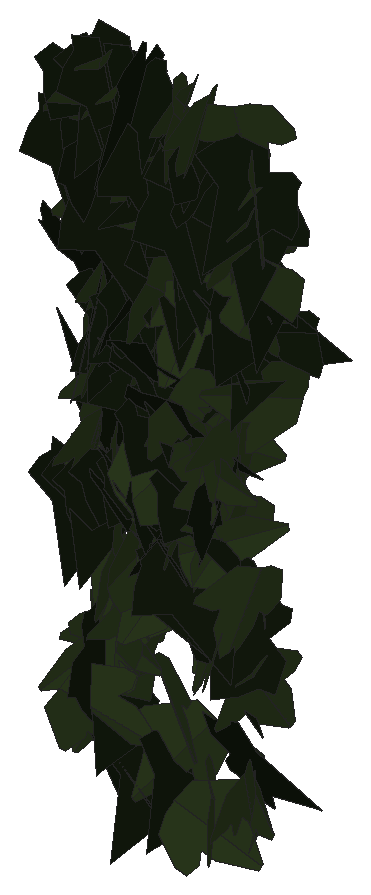
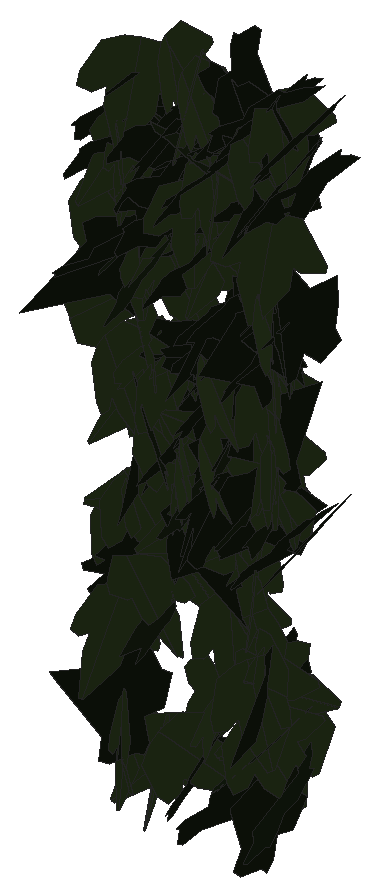
# SketchUp Ruby script. Lengths in inches.
U = 1.inch
M = Sketchup.active_model
def pt(a) = Geom::Point3d.new(a.map { |v| v * U })
def face(e, loops, mat)
  f = e.add_face(loops[0].map { |a| pt(a) })
  loops[1..].each { |l| e.add_face(l.map { |a| pt(a) }).erase! }
  f.material = f.back_material = mat if mat
  f
end
# faces: each face lists its corners as indices into pts; further lists are holes
def faces(e, pts, list, mat = nil) = list.each { |f| face(e, (f[0].is_a?(Array) ? f : [f]).map { |l| l.map { |i| pts[i] } }, mat) }
# xy, xz, yz: faces in a plane at the given z, y or x. An outline is a flat list of corners, or four numbers for a rectangle; further outlines are holes
def ring(l) = l.size == 4 ? [[l[0], l[1]], [l[2], l[1]], [l[2], l[3]], [l[0], l[3]]] : l.each_slice(2).to_a
def flat(e, list, mat, &to3) = list.each { |f| face(e, (f[0].is_a?(Array) ? f : [f]).map { |l| ring(l).map { |u, v| to3.(u, v) } }, mat) }
def xy(e, z, list, mat = nil) = flat(e, list, mat) { |x, y| [x, y, z] }
def xz(e, y, list, mat = nil) = flat(e, list, mat) { |x, z| [x, y, z] }
def yz(e, x, list, mat = nil) = flat(e, list, mat) { |y, z| [x, y, z] }
def lines(e, pts, list) = list.each { |a, b| e.add_line(pt(pts[a]), pt(pts[b])) }
# prism: a flat outline (further loops are holes) pulled along v
def prism(e, loops, v, mat = nil)
  f = face(e, loops, mat); d = Geom::Vector3d.new(v.map { |x| x * U })
  f.pushpull(f.normal.samedirection?(d) ? d.length : -d.length)
end
def box(e, o, s, mat = nil) = prism(e, [[o, [o[0] + s[0], o[1], o[2]], [o[0] + s[0], o[1] + s[1], o[2]], [o[0], o[1] + s[1], o[2]]]], [0, 0, s[2]], mat)
def at(x, y, z, deg = 0) = Geom::Transformation.translation(pt([x, y, z])) * Geom::Transformation.rotation(ORIGIN, Z_AXIS, deg.degrees)
def axes(o, x, y, z) = Geom::Transformation.new([*x, 0, *y, 0, *z, 0, *pt(o).to_a, 1])
def part(name) = M.definitions.add(name)
# library, detail: a bought-in or finely detailed component or shape, given as its bounding box
def library(name, o, s) = part(name).tap { |d| box(d.entities, o, s) }
def detail(e, o, s) = box(e.add_group.entities, o, s)
def put(e, d, t, mat = nil) = e.add_instance(d, t).tap { |i| i.material = mat if mat }
def group(e, t, mat = nil) = e.add_group.tap { |g| g.transformation = t; g.material = mat if mat }.entities
root = M.entities
M.materials.add("efeu1").color = [18, 25, 13]
M.materials.add("efeu2").color = [43, 57, 29]
c1 = part("ivyleaf_10")
p = [[0,0.5,-0.03],[-0.0625,2.02,-0.43],[-0.19,2.01,-0.46],[-0.54,1.05,-0.29],[-0.52,0.625,-0.18],[-0.83,0.76,-0.28],
  [-1.16,0.64,-0.33],[-1.15,0.33,-0.24],[-0.77,-0.39,0.02],[-0.3,-0.51,0.16],[0.04,-0.48,0.23],[-0.02,2.01,-0.4375],
  [-0.06,2.01,-0.43],[0.04,-0.49,0.23],[0.67,-0.49,0.14],[1.38,0.36,-0.2],[1.375,0.51,-0.24],[0.81,0.65,-0.19],
  [0.62,0.59,-0.15],[0.6,1.09,-0.28],[0.5,1.23,-0.31]]
faces(c1.entities,p,[[0,1,2,3,4,5,6,7,8,9,10],[11,12,0,13,14,15,16,17,18,19,20]],"efeu2")
c2 = part("ivyleaf_9")
p = [[1.54,2.16,1.25],[1.36,2.04,1.19],[-0.21,0.99,0.68],[-0.71,1.11,0.82],[-0.85,0.86,0.67],[-0.8,0.17,0.21],
  [-0.9,-0.01,0.1],[-0.67,-0.16,-0.02],[-0.08,-0.08,-0.05],[-0.03,-0.6,-0.4],[0.65,-0.88,-0.66],[0.83,-0.6,-0.49],
  [1.29,-0.42,-0.43],[1.8125,-0.07,-0.26],[1.21,0.44,0.15]]
faces(c2.entities,p,[[0,1,2,3,4,5,6,7,8,9,10,11,12,13,14]],"efeu1")
put(root,c1,axes([19.36,223.77,215.16],[-0.23772,-0.16251,-0.40876],[0.39056,0.13578,-0.28112],[0.20237,-0.45294,0.06239]))
put(root,c2,axes([21.28,224.3,220.56],[-0.0985,-0.38619,0.30192],[0.08114,-0.31655,-0.37843],[0.48344,-0.02556,0.12503]))
put(root,c2,axes([20.67,224.1,221.75],[0.00218,-0.49525,-0.06872],[0.00356,0.06873,-0.49524],[0.49998,0.00167,0.00383]))
put(root,c2,axes([19.62,223.89,217.87],[0.43761,-0.23745,-0.04594],[-0.03954,0.02345,-0.49788],[0.2386,0.43939,0.00174]))
put(root,c2,axes([20.26,223.86,219.03],[0.41406,-0.10025,0.26174],[0.25775,-0.04721,-0.42583],[0.11009,0.48757,0.01258]))
put(root,c2,axes([18.99,224.28,217.52],[-0.01258,-0.43972,0.23767],[0.03524,-0.23794,-0.43834],[0.4986,0.00572,0.03698]))
put(root,c1,axes([20.81,223.98,218.53],[-0.01124,-0.02847,0.49906],[0.49935,0.02224,0.01252],[-0.02291,0.49869,0.02793]))
put(root,c1,axes([19.6,223.86,219.81],[0.18106,-0.42203,-0.19777],[-0.04131,0.1968,-0.45778],[0.46423,0.18211,0.0364]))
put(root,c2,axes([19.66,224.04,221.51],[-0.01873,-0.4599,-0.19529],[0.07758,0.19038,-0.45578],[0.49359,-0.04737,0.06423]))
put(root,c2,axes([20.78,223.98,217.33],[-0.09563,-0.3888,-0.29948],[0.10782,0.28102,-0.39926],[0.47878,-0.14094,0.0301]))
put(root,c2,axes([19.76,224.1,217.92],[0.29761,-0.35976,0.17889],[0.118,-0.13453,-0.46688],[0.38406,0.32012,0.00483]))
put(root,c2,axes([19.8,223.87,219.47],[0.36058,-0.07558,0.33803],[0.33565,-0.04429,-0.36794],[0.08556,0.49227,0.0188]))
put(root,c1,axes([21.83,224.28,219.6],[-0.12293,-0.05949,-0.48099],[-0.32557,-0.35745,0.12742],[-0.35901,0.34452,0.04914]))
put(root,c2,axes([19.87,224.24,223.16],[-0.14768,0.10407,-0.46622],[0.34379,-0.31566,-0.17936],[-0.33166,-0.37354,0.02167]))
put(root,c1,axes([21.68,224.2,221.06],[-0.23682,-0.35163,0.26508],[-0.05351,-0.27578,-0.41362],[0.4371,-0.22428,0.09299]))
put(root,c1,axes([20.29,223.69,218.18],[0.23016,0.16438,-0.41232],[0.28106,0.30552,0.27869],[0.34356,-0.36006,0.04824]))
put(root,c1,axes([20.8,224.1,222.98],[0.11221,-0.4823,0.06923],[0.02283,-0.06576,-0.49513],[0.48671,0.11428,0.00726]))
put(root,c1,axes([20.98,223.73,214.24],[0.16554,0.27837,0.38093],[0.18768,0.33153,-0.32383],[-0.43287,0.2502,0.00528]))
put(root,c1,axes([21.49,224.15,217.17],[-0.11812,-0.45677,0.16556],[0.00814,-0.17222,-0.46933],[0.48578,-0.10818,0.04812]))
put(root,c1,axes([20.9,224.28,218.4],[0.004,-0.36862,0.33779],[0.00435,-0.33777,-0.36864],[0.49997,0.00589,0.0005]))
put(root,c2,axes([20.36,224.39,214.26],[-0.02165,-0.35434,0.3521],[-0.03301,-0.35064,-0.35491],[0.49844,-0.03861,-0.00821]))
put(root,c1,axes([21.08,223.99,216.51],[0.30073,-0.37516,-0.13719],[-0.08719,0.10594,-0.48081],[0.38982,0.31311,-0.0017]))
put(root,c1,axes([20.07,223.66,217.01],[0.0548,-0.12882,0.48],[-0.16891,0.44934,0.13987],[-0.4674,-0.17749,0.00573]))
put(root,c2,axes([19.99,224.09,222.31],[0.09641,-0.46121,-0.1673],[-0.04194,0.16213,-0.47112],[0.48882,0.10487,-0.00742]))
put(root,c1,axes([20.35,224.09,216.94],[0.43665,0.10375,-0.2204],[-0.21642,-0.04243,-0.44873],[-0.11182,0.48727,0.00785]))
put(root,c1,axes([20.75,223.8,219.37],[-0.13643,-0.33324,-0.3469],[0.18864,0.29463,-0.35722],[0.44249,-0.22835,0.04533]))
put(root,c2,axes([20.22,223.99,219],[0.23141,-0.38588,-0.21805],[-0.06878,0.21173,-0.4477],[0.43786,0.2372,0.04492]))
put(root,c2,axes([21.49,224.4,222.29],[-0.18047,-0.41727,0.20812],[-0.06632,-0.19793,-0.45434],[0.46155,-0.1916,0.0161]))
put(root,c2,axes([19.28,224.2,220.34],[-0.26118,0.12892,-0.4064],[0.37718,-0.15236,-0.29073],[-0.1988,-0.45844,-0.01766]))
put(root,c1,axes([19.53,224.14,219.25],[-0.07199,-0.4882,0.08048],[-0.01316,-0.0794,-0.49348],[0.49462,-0.07317,-0.00142]))
put(root,c1,axes([21.54,223.96,221.74],[0.01716,-0.469,-0.17246],[0.02403,0.17314,-0.46845],[0.49913,0.00779,0.02848]))
put(root,c2,axes([21.51,224.33,216.43],[-0.16723,-0.38205,-0.27582],[-0.08297,-0.26423,0.41629],[-0.46384,0.185,0.02498]))
put(root,c2,axes([20.68,224.24,219.48],[-0.38663,-0.03855,0.31469],[-0.30971,-0.06021,-0.38788],[0.0678,-0.49486,0.02268]))
put(root,c1,axes([19.4375,224.29,215.76],[0.13641,0.21483,-0.4304],[-0.28951,-0.32061,-0.25178],[-0.38416,0.3179,0.03692]))
put(root,c1,axes([20.36,223.78,220.76],[-0.02404,-0.31504,-0.38752],[0.0435,0.38517,-0.31583],[0.49752,-0.0489,0.0089]))
put(root,c1,axes([19.31,224.11,218.5],[0.04101,-0.49818,-0.01178],[-0.00408,0.01149,-0.49985],[0.4983,0.0411,-0.00312]))
put(root,c2,axes([18.95,224.28,222.09],[-0.00324,-0.49991,-0.0088],[-0.00007,0.0088,-0.49992],[0.49999,-0.00324,-0.00012]))
put(root,c1,axes([19.72,223.89,217.03],[0.14313,-0.38679,-0.28267],[0.00895,0.29713,-0.40204],[0.47899,0.11003,0.09198]))
put(root,c1,axes([21.36,224.02,219.2],[-0.09817,-0.47753,-0.11103],[0.02174,0.10889,-0.48751],[0.48979,-0.10054,-0.00062]))
put(root,c1,axes([20.8,224.18,218.99],[-0.15412,-0.46684,0.09117],[-0.01713,-0.09032,-0.49148],[0.47535,-0.15461,0.01184]))
put(root,c2,axes([19.97,224.33,219.63],[0.10588,-0.47899,0.09673],[0.02629,-0.09325,-0.49052],[0.48795,0.10896,0.00544]))
put(root,c1,axes([21.01,224.29,217.77],[-0.04092,-0.45785,0.19673],[0.0434,-0.19992,-0.45623],[0.49643,-0.02026,0.0561]))
put(root,c2,axes([19.38,223.8,222.25],[0.1402,-0.06128,-0.47601],[-0.28478,0.38855,-0.1339],[0.38632,0.30866,0.07404]))
put(root,c2,axes([19.53,224.05,218.51],[0.13589,-0.20459,0.43552],[-0.23921,0.36395,0.2456],[-0.41751,-0.27511,0.00103]))
put(root,c2,axes([20.65,224.09,218.27],[0.20615,-0.39177,-0.23241],[-0.08698,0.21656,-0.4422],[0.44714,0.22275,0.02113]))
put(root,c2,axes([19.16,224.46,217.57],[-0.06949,-0.46554,0.16865],[0.02645,-0.17355,-0.46817],[0.49444,-0.05615,0.04875]))
put(root,c1,axes([19.98,224.14,216.37],[-0.17637,-0.46748,-0.01892],[0.0029,0.01913,-0.49963],[0.46785,-0.17634,-0.00404]))
put(root,c2,axes([20.68,224.27,222.14],[-0.47046,0.16918,-0.00681],[-0.04142,-0.13452,-0.47978],[-0.16417,-0.45087,0.14059]))
put(root,c1,axes([20.66,224.1875,220.41],[0.42817,0.21561,-0.14206],[-0.1375,-0.04246,-0.47884],[-0.21855,0.44912,0.02293]))
put(root,c2,axes([19.89,224.17,220.17],[0.02434,-0.4358,-0.2439],[0.00026,0.2442,-0.43631],[0.49941,0.02111,0.01212]))
put(root,c2,axes([21.43,224.47,221.06],[0.06612,-0.43025,0.24599],[0.01721,-0.24603,-0.43494],[0.49531,0.06599,-0.01773]))
put(root,c2,axes([19.39,224.51,219.85],[-0.05892,-0.42412,0.25816],[-0.01141,-0.25875,-0.42769],[0.49639,-0.05629,0.02081]))
put(root,c2,axes([20.39,224.17,217.48],[-0.18987,0.39838,-0.23504],[0.10745,-0.20913,-0.44127],[-0.4499,-0.21807,-0.0062]))
put(root,c2,axes([19.32,224.38,222.91],[0.03674,-0.49838,0.01634],[0.00149,-0.01628,-0.49973],[0.49865,0.03677,0.00029]))
put(root,c2,axes([19.77,224.28,223],[-0.36886,-0.1246,-0.31372],[0.28958,0.12199,-0.38893],[0.17346,-0.46861,-0.01783]))
put(root,c2,axes([21.11,223.88,218.47],[0.06993,-0.06188,-0.4912],[-0.35335,0.34123,-0.09329],[0.34677,0.36018,0.004]))
put(root,c1,axes([19.32,224.33,220.38],[0.14411,-0.46246,0.12394],[0.04268,-0.11651,-0.48436],[0.47688,0.15018,0.00589]))
put(root,c2,axes([21.38,224.44,221.9375],[-0.0742,-0.49431,0.0122],[-0.00148,-0.01212,-0.49985],[0.49446,-0.07421,0.00033]))
put(root,c2,axes([19.42,223.82,215.8],[0.07062,0.06291,-0.49097],[-0.34984,0.35719,-0.00455],[0.35017,0.34417,0.09446]))
put(root,c2,axes([19.8125,224.3,219.78],[-0.17401,-0.41337,-0.221],[0.08339,0.20468,-0.4485],[0.46127,-0.19295,-0.00229]))
put(root,c1,axes([19.41,224.29,216.67],[0.27488,-0.03656,0.41606],[0.41008,-0.07085,-0.27715],[0.07922,0.4936,-0.00897]))
put(root,c1,axes([19.45,224.25,218.49],[-0.36035,0.26623,-0.22196],[0.13341,-0.18899,-0.44327],[-0.31992,-0.37869,0.06518]))
put(root,c2,axes([19.45,224.53,222.875],[-0.20913,-0.43499,0.13056],[-0.02625,-0.13192,-0.48157],[0.4534,-0.20828,0.03235]))
put(root,c2,axes([19.4,224.57,214.91],[-0.10179,-0.4027,0.27834],[0.06493,-0.29289,-0.4],[0.4852,-0.04529,0.11192]))
put(root,c1,axes([19.5,224.09,218.74],[0.35416,-0.28105,-0.21351],[-0.08105,0.22962,-0.4367],[0.34351,0.34393,0.11708]))
put(root,c2,axes([20.76,224.42,222.29],[-0.11636,-0.48408,-0.04612],[0.00535,0.04615,-0.49784],[0.48624,-0.11635,-0.00556]))
put(root,c1,axes([21.375,224.13,220.69],[-0.45441,0.06146,0.19934],[-0.19993,0.00801,-0.45822],[-0.05951,-0.49614,0.01729]))
put(root,c1,axes([19.4,224.39,215.15],[-0.22259,-0.37524,0.24423],[-0.08911,-0.23015,-0.43484],[0.43876,-0.23711,0.03558]))
put(root,c1,axes([19.21,224.23,222.87],[-0.08937,-0.49119,-0.02729],[0.00618,0.02661,-0.49925],[0.49191,-0.08958,0.00132]))
put(root,c1,axes([21.28,224.14,219.82],[0.34647,-0.29149,-0.21212],[-0.11981,0.18437,-0.44906],[0.34001,0.362,0.05791]))
put(root,c2,axes([18.76,224.43,220.23],[-0.04881,-0.14926,0.4747],[0.31668,-0.37724,-0.08605],[0.38384,0.29226,0.13136]))
put(root,c2,axes([21.11,224.3125,214.8],[0.26116,-0.17413,0.3892],[0.31746,-0.22526,-0.3138],[0.28463,0.41102,-0.0071]))
put(root,c2,axes([19.91,224.58,214.2],[-0.14,-0.43473,0.2035],[-0.05844,-0.19496,-0.4567],[0.47643,-0.15166,0.00378]))
put(root,c1,axes([21.39,224.12,214.6],[0.05343,-0.45503,-0.20024],[0.02658,0.20372,-0.45584],[0.49643,0.03807,0.04596]))
put(root,c1,axes([20.54,224.3,216.99],[0.43773,0.09448,-0.22241],[-0.21703,-0.04864,-0.44781],[-0.10626,0.48858,-0.00157]))
put(root,c2,axes([20.12,224.01,218.18],[0.21405,-0.17996,-0.41448],[-0.30023,0.28612,-0.27927],[0.3377,0.36844,0.01443]))
put(root,c1,axes([21.04,223.99,214.35],[0.20972,-0.2827,-0.35511],[-0.04387,0.37672,-0.32581],[0.45177,0.16782,0.13321]))
put(root,c2,axes([19.73,223.82,219.72],[0.07295,0.20088,0.45202],[0.13563,0.43128,-0.21355],[-0.47569,0.15378,0.00843]))
put(root,c2,axes([19.71,224.0625,218.22],[-0.03357,-0.09632,-0.48949],[0.21802,0.43843,-0.10122],[0.44871,-0.22023,0.01257]))
put(root,c1,axes([20.4375,224.28,218.19],[0.19434,-0.45828,-0.04702],[-0.02174,0.04186,-0.49777],[0.46017,0.19552,-0.00365]))
put(root,c1,axes([20.32,224.39,222.83],[0.15086,-0.46608,0.10003],[0.02546,-0.09689,-0.48986],[0.47602,0.1529,-0.0055]))
put(root,c1,axes([21.48,224,221.82],[-0.1085,-0.30576,-0.38045],[0.14489,0.35199,-0.32421],[0.46608,-0.1806,0.01223]))
put(root,c2,axes([21.5625,224.58,220.41],[-0.21624,-0.43956,0.10016],[-0.00504,-0.10872,-0.48801],[0.45079,-0.21206,0.04259]))
put(root,c1,axes([19.45,224.47,222.49],[0.04592,-0.44532,0.22266],[0.01349,-0.22241,-0.44761],[0.4977,0.04711,-0.00842]))
put(root,c1,axes([19.27,224.2,218.11],[0.33985,0.13892,0.33942],[0.31755,0.12006,-0.36708],[-0.18349,0.46507,-0.00663]))
put(root,c1,axes([20.42,224.54,214.74],[-0.21002,-0.24361,0.38281],[-0.11529,-0.37934,-0.30465],[0.43886,-0.21624,0.10317]))
put(root,c1,axes([21.2,224.46,214.31],[-0.0132,0.0171,0.49953],[0.45614,-0.2039,0.01903],[0.20436,0.45622,-0.01022]))
put(root,c2,axes([20.58,224.31,221.69],[0.03754,-0.44103,-0.23257],[-0.01988,0.23171,-0.44262],[0.49819,0.04248,-0.00013]))
put(root,c2,axes([20.65,224.33,216.36],[0.33134,-0.37397,-0.01897],[-0.01196,0.01475,-0.49964],[0.37426,0.33155,0.00082]))
put(root,c1,axes([20.49,224.04,222.82],[0.14556,-0.32253,-0.35325],[0.00858,0.37094,-0.33515],[0.47827,0.09151,0.11352]))
put(root,c1,axes([19.4,224.23,221.3],[-0.44255,-0.22914,-0.04058],[0.03601,0.01871,-0.49835],[0.2299,-0.44401,-0.00006]))
put(root,c2,axes([20.63,224.5625,221.27],[-0.15035,-0.47431,0.04921],[-0.02516,-0.04364,-0.49746],[0.47619,-0.15206,-0.01074]))
put(root,c1,axes([21.25,224.5,222.1],[0.17524,-0.25089,0.3954],[0.35489,-0.20429,-0.28691],[0.30552,0.38121,0.10648]))
put(root,c2,axes([20.89,224.57,220.41],[0.12721,-0.41937,0.24072],[0.07712,-0.22813,-0.43819],[0.47736,0.14861,0.00664]))
put(root,c1,axes([20.15,224.3125,221.65],[-0.33434,0.3375,-0.15592],[0.06844,-0.15024,-0.47196],[-0.36542,-0.33693,0.05427]))
put(root,c2,axes([19.09,224.51,214.13],[0.1776,-0.27408,0.3786],[0.24005,-0.29403,-0.32546],[0.40104,0.29737,0.02715]))
put(root,c1,axes([19.21,224.34,215.78],[0.04489,-0.01857,0.49763],[0.49798,0.00181,-0.04485],[-0.00013,0.49965,0.01866]))
put(root,c2,axes([19.45,224.14,218.01],[-0.00116,-0.19951,-0.45847],[0.11978,0.44501,-0.19396],[0.48544,-0.11028,0.04676]))
put(root,c1,axes([20.9375,223.97,217.49],[-0.01334,-0.07114,0.49473],[0.13978,0.47463,0.07202],[-0.47988,0.14023,0.00722]))
put(root,c2,axes([20.92,224.47,218.7],[-0.32396,0.09817,-0.36798],[0.35396,-0.1007,-0.33849],[-0.14057,-0.47981,-0.00425]))
put(root,c1,axes([20.36,224.44,218.08],[0.17378,-0.46311,0.07303],[0.04808,-0.05987,-0.49407],[0.46636,0.17874,0.02373]))
put(root,c2,axes([18.83,224.34,222.82],[0.23346,-0.41492,-0.15275],[-0.0131,0.16617,-0.4714],[0.44195,0.22411,0.06672]))
put(root,c1,axes([19.98,224.48,219.5],[0.1498,-0.46225,0.11782],[0.02743,-0.11494,-0.48584],[0.47624,0.15202,-0.00908]))
put(root,c2,axes([20.19,224.59,220.84],[-0.00597,-0.49796,0.04476],[0.00365,-0.04481,-0.49797],[0.49995,-0.00562,0.00417]))
put(root,c1,axes([20.07,224.36,221.9375],[-0.08328,-0.49246,-0.02338],[-0.00044,0.02379,-0.49943],[0.49301,-0.08317,-0.0044]))
put(root,c1,axes([20.33,224.33,221.51],[-0.33953,-0.36695,-0.0081],[0.00702,0.00454,-0.49993],[0.36697,-0.3396,0.00207]))
put(root,c1,axes([20.56,224.19,217.8125],[0.10038,-0.41424,-0.2614],[0.00458,0.26761,-0.42233],[0.4898,0.08239,0.05752]))
put(root,c1,axes([21.18,224.08,218.93],[-0.0148,-0.28772,-0.40865],[0.17245,0.38079,-0.27434],[0.46909,-0.14906,0.08796]))
put(root,c2,axes([18.9,224.61,214.48],[0.19087,-0.39923,0.23278],[0.10402,-0.20827,-0.4425],[0.45028,0.21734,0.00355]))
put(root,c1,axes([20.08,224.39,215.43],[-0.32172,0.30109,-0.23631],[0.18407,-0.14894,-0.44038],[-0.33558,-0.37035,-0.01501]))
put(root,c1,axes([20.97,224.57,217.73],[-0.21891,-0.38324,0.23496],[-0.01495,-0.25499,-0.42984],[0.44928,-0.19522,0.10018]))
put(root,c2,axes([18.99,224.47,222.22],[0.21069,-0.44942,-0.06029],[-0.02067,0.05689,-0.49632],[0.45297,0.21163,0.00539]))
put(root,c2,axes([20.54,224.36,222.375],[0.24063,-0.39779,-0.184],[-0.06632,0.17444,-0.46386],[0.43324,0.24765,0.03119]))
put(root,c2,axes([20.04,224.66,218.04],[0.11664,-0.39312,0.2861],[0.1319,-0.2576,-0.40773],[0.46797,0.17059,0.04361]))
put(root,c2,axes([20.03,224.58,221.96],[0.06458,-0.49564,0.01317],[0.00157,-0.01308,-0.49983],[0.49581,0.0646,-0.00013]))
put(root,c1,axes([21.17,224.33,222.9],[-0.43707,-0.23875,-0.04439],[0.03897,0.02125,-0.49803],[0.23969,-0.4388,0.00003]))
put(root,c1,axes([21.03,224.4,216.61],[0.46507,-0.02538,-0.18183],[-0.17962,0.03956,-0.46494],[0.03798,0.49779,0.02768]))
put(root,c2,axes([19.77,224.28,220.32],[0.20432,-0.33645,-0.30831],[-0.08804,0.30239,-0.38834],[0.44777,0.21299,0.06433]))
put(root,c1,axes([19.92,224.57,218.53],[0.18638,-0.4358,0.1592],[0.06908,-0.14358,-0.47393],[0.45879,0.19866,0.00669]))
put(root,c1,axes([19.42,224.47,215.84],[-0.25119,-0.42273,0.09057],[-0.03894,-0.0822,-0.49166],[0.43057,-0.25405,0.00838]))
put(root,c1,axes([21.51,224.23,215.92],[-0.15339,-0.39619,-0.26363],[0.09004,0.24782,-0.42483],[0.46729,-0.1778,-0.00468]))
put(root,c1,axes([21.29,224.52,219.26],[0.03362,-0.49025,0.09232],[-0.00877,-0.09309,-0.49118],[0.49879,0.0314,-0.01486]))
put(root,c2,axes([21.34,224.07,220.43],[0.11351,-0.00301,-0.48694],[-0.01175,0.49983,-0.00583],[0.4868,0.01277,0.1134]))
put(root,c2,axes([20.51,224.66,221.84],[-0.17845,-0.46707,0.00021],[-0.00299,0.00092,-0.49999],[0.46706,-0.17844,-0.00312]))
put(root,c1,axes([20.18,224.13,217.66],[-0.13169,-0.16487,-0.45329],[0.30246,0.3378,-0.21073],[0.37573,-0.32971,0.01076]))
put(root,c2,axes([19.79,224.34,218.13],[0.11497,-0.36909,-0.3171],[-0.07602,0.30821,-0.3863],[0.48063,0.13704,0.01475]))
